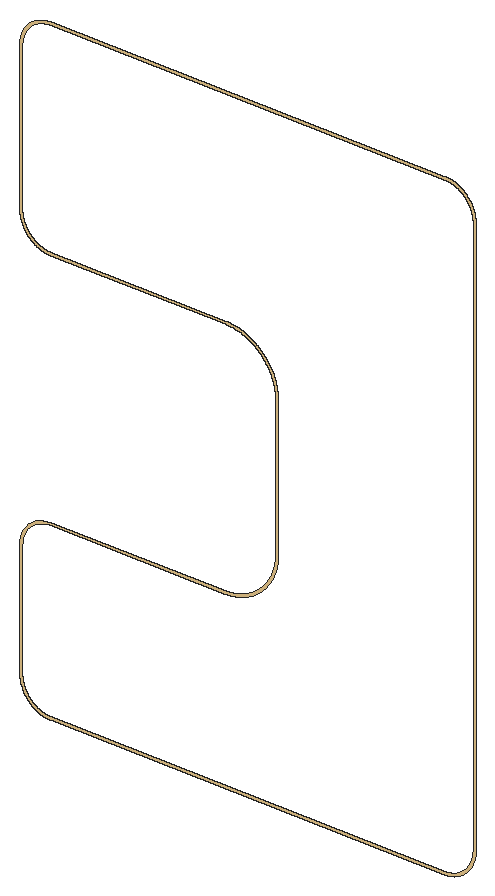
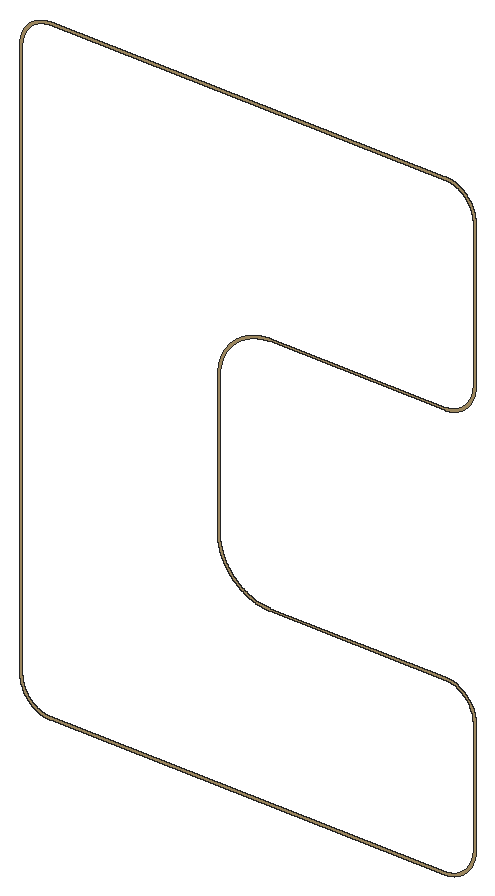
# SketchUp Ruby script. Lengths in inches.
U = 1.inch
M = Sketchup.active_model
def pt(a) = Geom::Point3d.new(a.map { |v| v * U })
def face(e, loops, mat)
  f = e.add_face(loops[0].map { |a| pt(a) })
  loops[1..].each { |l| e.add_face(l.map { |a| pt(a) }).erase! }
  f.material = f.back_material = mat if mat
  f
end
# faces: each face lists its corners as indices into pts; further lists are holes
def faces(e, pts, list, mat = nil) = list.each { |f| face(e, (f[0].is_a?(Array) ? f : [f]).map { |l| l.map { |i| pts[i] } }, mat) }
# xy, xz, yz: faces in a plane at the given z, y or x. An outline is a flat list of corners, or four numbers for a rectangle; further outlines are holes
def ring(l) = l.size == 4 ? [[l[0], l[1]], [l[2], l[1]], [l[2], l[3]], [l[0], l[3]]] : l.each_slice(2).to_a
def flat(e, list, mat, &to3) = list.each { |f| face(e, (f[0].is_a?(Array) ? f : [f]).map { |l| ring(l).map { |u, v| to3.(u, v) } }, mat) }
def xy(e, z, list, mat = nil) = flat(e, list, mat) { |x, y| [x, y, z] }
def xz(e, y, list, mat = nil) = flat(e, list, mat) { |x, z| [x, y, z] }
def yz(e, x, list, mat = nil) = flat(e, list, mat) { |y, z| [x, y, z] }
def lines(e, pts, list) = list.each { |a, b| e.add_line(pt(pts[a]), pt(pts[b])) }
# prism: a flat outline (further loops are holes) pulled along v
def prism(e, loops, v, mat = nil)
  f = face(e, loops, mat); d = Geom::Vector3d.new(v.map { |x| x * U })
  f.pushpull(f.normal.samedirection?(d) ? d.length : -d.length)
end
def box(e, o, s, mat = nil) = prism(e, [[o, [o[0] + s[0], o[1], o[2]], [o[0] + s[0], o[1] + s[1], o[2]], [o[0], o[1] + s[1], o[2]]]], [0, 0, s[2]], mat)
def at(x, y, z, deg = 0) = Geom::Transformation.translation(pt([x, y, z])) * Geom::Transformation.rotation(ORIGIN, Z_AXIS, deg.degrees)
def axes(o, x, y, z) = Geom::Transformation.new([*x, 0, *y, 0, *z, 0, *pt(o).to_a, 1])
def part(name) = M.definitions.add(name)
# library, detail: a bought-in or finely detailed component or shape, given as its bounding box
def library(name, o, s) = part(name).tap { |d| box(d.entities, o, s) }
def detail(e, o, s) = box(e.add_group.entities, o, s)
def put(e, d, t, mat = nil) = e.add_instance(d, t).tap { |i| i.material = mat if mat }
def group(e, t, mat = nil) = e.add_group.tap { |g| g.transformation = t; g.material = mat if mat }.entities
root = M.entities
M.materials.add("Outer Light").color = [251, 217, 152]
xz(root,95.37,[[[278.68,171.29,537.32,171.29,537.48,171.3,537.64,171.3,537.8,171.31,537.97,171.31,538.125,171.32,538.29,171.33,538.45,171.34,538.61,171.36,538.93,171.38,539.25,171.42,539.41,171.43,539.73,171.47,539.89,171.5,540.21,171.54,540.37,171.57,540.52,171.6,540.68,171.625,540.84,171.66,541,171.6875,541.16,171.72,541.31,171.75,541.47,171.79,541.63,171.82,541.79,171.86,541.94,171.9,542.1,171.9375,542.25,171.98,542.41,172.02,542.56,172.0625,542.72,172.11,542.875,172.15,543.03,172.2,543.33,172.3,543.49,172.35,543.94,172.5,544.1,172.56,544.25,172.62,544.4,172.67,544.85,172.85,544.99,172.91,545.14,172.98,545.29,173.04,545.4375,173.11,545.58,173.18,545.73,173.24,545.875,173.3125,546.02,173.38,546.16,173.45,546.31,173.53,546.59,173.67,546.73,173.75,547.02,173.91,547.44,174.15,547.57,174.23,547.71,174.3125,547.85,174.4,547.98,174.48,548.12,174.57,548.25,174.66,548.39,174.75,548.52,174.84,548.66,174.93,548.92,175.11,549.05,175.21,549.18,175.3,549.31,175.4,549.4375,175.5,549.56,175.59,549.82,175.79,549.94,175.89,550.07,176,550.19,176.1,550.3125,176.2,550.4375,176.31,550.56,176.41,550.92,176.74,551.03,176.85,551.27,177.07,551.61,177.41,551.72,177.53,551.83,177.64,551.94,177.76,552.05,177.875,552.16,178,552.27,178.11,552.38,178.24,552.48,178.36,552.59,178.48,552.69,178.6,552.8,178.72,552.9,178.85,553,178.97,553.3,179.36,553.39,179.48,553.49,179.61,553.58,179.74,553.68,179.875,553.77,180,553.86,180.14,553.96,180.27,554.05,180.4,554.13,180.54,554.22,180.67,554.31,180.81,554.39,180.94,554.48,181.08,554.5625,181.22,554.65,181.36,554.89,181.78,554.96,181.92,555.12,182.2,555.19,182.34,555.27,182.49,555.41,182.77,555.48,182.92,555.55,183.0625,555.62,183.21,555.68,183.36,555.75,183.5,555.8125,183.65,555.88,183.8,556.18,184.55,556.23,184.7,556.29,184.85,556.39,185.15,556.45,185.3,556.5,185.46,556.55,185.61,556.59,185.76,556.64,185.92,556.6875,186.07,556.73,186.23,556.77,186.38,556.82,186.54,556.86,186.69,556.9,186.85,556.93,187.01,556.97,187.16,557.01,187.32,557.04,187.48,557.07,187.63,557.11,187.79,557.17,188.11,557.19,188.27,557.25,188.59,557.27,188.74,557.3,188.9,557.32,189.0625,557.34,189.22,557.36,189.38,557.39,189.7,557.41,189.86,557.42,190.02,557.4375,190.18,557.45,190.34,557.46,190.5,557.47,190.67,557.48,190.83,557.48,190.99,557.49,191.15,557.49,191.31,557.5,191.47,557.5,561.11,557.49,561.28,557.49,561.4375,557.48,561.6,557.48,561.76,557.45,562.24,557.4375,562.4,557.42,562.5625,557.41,562.72,557.39,562.88,557.36,563.2,557.3,563.68,557.27,563.84,557.25,564,557.19,564.32,557.17,564.48,557.14,564.63,557.11,564.79,557.07,564.95,557.04,565.11,557.01,565.26,556.93,565.58,556.9,565.73,556.82,566.05,556.77,566.2,556.73,566.36,556.6875,566.51,556.64,566.67,556.59,566.82,556.55,566.97,556.45,567.28,556.39,567.43,556.34,567.58,556.29,567.74,556.23,567.89,556.18,568.04,556.12,568.1875,556.06,568.34,555.88,568.79,555.8125,568.93,555.75,569.08,555.68,569.23,555.62,569.375,555.55,569.52,555.48,569.67,555.41,569.8125,555.34,569.96,555.27,570.1,555.19,570.24,555.12,570.38,555.04,570.53,554.96,570.67,554.89,570.81,554.65,571.23,554.5625,571.37,554.48,571.5,554.39,571.64,554.31,571.78,554.22,571.91,554.13,572.05,554.05,572.18,553.96,572.31,553.86,572.45,553.68,572.71,553.58,572.84,553.49,572.97,553.39,573.1,553.3,573.23,553.2,573.36,553.1,573.48,553,573.61,552.9,573.73,552.8,573.86,552.69,573.98,552.59,574.11,552.48,574.23,552.38,574.35,551.94,574.83,551.83,574.94,551.72,575.06,551.61,575.17,551.5,575.29,551.38,575.4,551.27,575.51,551.03,575.74,550.92,575.85,550.8,575.95,550.68,576.0625,550.56,576.17,550.4375,576.28,550.3125,576.38,550.19,576.48,550.07,576.59,549.94,576.69,549.82,576.79,549.56,576.99,549.4375,577.09,549.31,577.1875,549.18,577.28,548.92,577.47,548.79,577.5625,548.66,577.66,548.52,577.75,548.39,577.84,548.25,577.93,548.12,578.01,547.98,578.1,547.85,578.1875,547.71,578.27,547.57,578.35,547.44,578.4375,547.3,578.52,547.02,578.68,546.875,578.76,546.73,578.83,546.59,578.91,546.45,578.98,546.31,579.06,546.16,579.13,546.02,579.2,545.73,579.34,545.58,579.41,545.4375,579.48,545.29,579.54,545.14,579.61,544.99,579.67,544.85,579.73,544.25,579.97,544.1,580.02,543.94,580.08,543.79,580.13,543.64,580.1875,543.49,580.24,543.33,580.29,543.03,580.39,542.875,580.43,542.72,580.48,542.56,580.52,542.41,580.57,542.25,580.61,542.1,580.65,541.94,580.6875,541.79,580.73,541.63,580.76,541.47,580.8,541.31,580.83,541.16,580.87,540.52,580.99,540.37,581.01,540.21,581.04,540.05,581.0625,539.89,581.09,539.09,581.19,538.93,581.2,538.77,581.22,538.29,581.25,538.125,581.26,537.97,581.27,537.8,581.28,537.64,581.28,537.48,581.29,278.52,581.29,278.36,581.28,278.2,581.28,278.03,581.27,277.875,581.26,277.71,581.25,277.23,581.22,277.07,581.2,276.91,581.19,276.11,581.09,275.95,581.0625,275.79,581.04,275.63,581.01,275.48,580.99,274.84,580.87,274.69,580.83,274.53,580.8,274.37,580.76,274.21,580.73,274.06,580.6875,273.9,580.65,273.75,580.61,273.59,580.57,273.44,580.52,273.28,580.48,273.125,580.43,272.97,580.39,272.67,580.29,272.51,580.24,272.36,580.1875,272.21,580.13,272.06,580.08,271.9,580.02,271.75,579.97,271.15,579.73,271.01,579.67,270.86,579.61,270.71,579.54,270.5625,579.48,270.42,579.41,270.27,579.34,269.98,579.2,269.84,579.13,269.69,579.06,269.55,578.98,269.41,578.91,269.27,578.83,269.125,578.76,268.98,578.68,268.7,578.52,268.56,578.4375,268.43,578.35,268.29,578.27,268.15,578.1875,268.02,578.1,267.88,578.01,267.75,577.93,267.61,577.84,267.48,577.75,267.34,577.66,267.21,577.5625,267.08,577.47,266.82,577.28,266.69,577.1875,266.5625,577.09,266.44,576.99,266.18,576.79,266.06,576.69,265.93,576.59,265.81,576.48,265.6875,576.38,265.5625,576.28,265.44,576.17,265.32,576.0625,265.2,575.95,265.08,575.85,264.97,575.74,264.73,575.51,264.62,575.4,264.5,575.29,264.39,575.17,264.28,575.06,264.17,574.94,264.06,574.83,263.62,574.35,263.52,574.23,263.41,574.11,263.31,573.98,263.2,573.86,263.1,573.73,263,573.61,262.9,573.48,262.8,573.36,262.7,573.23,262.61,573.1,262.51,572.97,262.42,572.84,262.32,572.71,262.14,572.45,262.04,572.31,261.95,572.18,261.87,572.05,261.78,571.91,261.69,571.78,261.61,571.64,261.52,571.5,261.4375,571.37,261.35,571.23,261.11,570.81,261.04,570.67,260.96,570.53,260.88,570.38,260.81,570.24,260.73,570.1,260.66,569.96,260.59,569.8125,260.52,569.67,260.45,569.52,260.38,569.375,260.32,569.23,260.25,569.08,260.1875,568.93,260.12,568.79,259.94,568.34,259.88,568.1875,259.82,568.04,259.77,567.89,259.71,567.74,259.66,567.58,259.61,567.43,259.55,567.28,259.45,566.97,259.41,566.82,259.36,566.67,259.3125,566.51,259.27,566.36,259.23,566.2,259.18,566.05,259.1,565.73,259.07,565.58,258.99,565.26,258.96,565.11,258.93,564.95,258.89,564.79,258.86,564.63,258.83,564.48,258.81,564.32,258.75,564,258.73,563.84,258.7,563.68,258.64,563.2,258.61,562.88,258.59,562.72,258.58,562.5625,258.5625,562.4,258.55,562.24,258.52,561.76,258.52,561.6,258.51,561.4375,258.51,561.28,258.5,561.11,258.5,464.47,258.51,464.31,258.51,464.15,258.52,463.99,258.52,463.83,258.53,463.67,258.54,463.5,258.55,463.34,258.5625,463.18,258.58,463.02,258.59,462.86,258.61,462.7,258.64,462.38,258.66,462.22,258.68,462.0625,258.7,461.9,258.73,461.74,258.75,461.59,258.81,461.27,258.83,461.11,258.89,460.79,258.93,460.63,258.96,460.48,258.99,460.32,259.03,460.16,259.07,460.01,259.1,459.85,259.14,459.69,259.18,459.54,259.23,459.38,259.27,459.23,259.3125,459.07,259.36,458.92,259.41,458.76,259.45,458.61,259.5,458.46,259.55,458.3,259.61,458.15,259.71,457.85,259.77,457.7,259.82,457.55,260.12,456.8,260.1875,456.65,260.25,456.5,260.32,456.36,260.38,456.21,260.45,456.0625,260.52,455.92,260.59,455.77,260.73,455.49,260.81,455.34,260.88,455.2,261.04,454.92,261.11,454.78,261.35,454.36,261.4375,454.22,261.52,454.08,261.61,453.94,261.69,453.81,261.78,453.67,261.87,453.54,261.95,453.4,262.04,453.27,262.14,453.14,262.23,453,262.32,452.875,262.42,452.74,262.51,452.61,262.61,452.48,262.7,452.36,263,451.97,263.1,451.85,263.2,451.72,263.31,451.6,263.41,451.48,263.52,451.36,263.62,451.24,263.73,451.11,263.84,451,263.95,450.875,264.06,450.76,264.17,450.64,264.28,450.53,264.39,450.41,264.73,450.07,264.97,449.85,265.08,449.74,265.44,449.41,265.5625,449.31,265.6875,449.2,265.81,449.1,265.93,449,266.06,448.89,266.18,448.79,266.44,448.59,266.5625,448.5,266.69,448.4,266.82,448.3,266.95,448.21,267.08,448.11,267.34,447.93,267.48,447.84,267.61,447.75,267.75,447.66,267.88,447.57,268.02,447.48,268.15,447.4,268.29,447.3125,268.43,447.23,268.56,447.15,268.98,446.91,269.27,446.75,269.41,446.67,269.69,446.53,269.84,446.45,269.98,446.38,270.125,446.3125,270.27,446.24,270.42,446.18,270.5625,446.11,270.71,446.04,270.86,445.98,271.01,445.91,271.15,445.85,271.6,445.67,271.75,445.62,271.9,445.56,272.06,445.5,272.51,445.35,272.67,445.3,272.97,445.2,273.125,445.15,273.28,445.11,273.44,445.0625,273.59,445.02,273.75,444.98,273.9,444.9375,274.06,444.9,274.21,444.86,274.37,444.82,274.53,444.79,274.69,444.75,274.84,444.72,275,444.6875,275.16,444.66,275.32,444.625,275.48,444.6,275.63,444.57,275.79,444.54,276.11,444.5,276.27,444.47,276.59,444.43,276.75,444.42,277.07,444.38,277.39,444.36,277.55,444.34,277.71,444.33,277.875,444.32,278.03,444.31,278.2,444.31,278.36,444.3,278.52,444.3,278.68,444.29,393.4375,444.29,393.875,444.28,394.32,444.27,394.75,444.25,395.19,444.22,395.63,444.1875,396.07,444.15,396.5,444.11,396.9375,444.06,397.37,444.01,397.81,443.95,398.67,443.81,399.1,443.73,399.54,443.65,399.97,443.56,400.39,443.47,400.82,443.37,401.25,443.26,401.67,443.15,402.93,442.79,403.77,442.51,404.18,442.37,404.59,442.22,405.01,442.07,405.41,441.91,405.82,441.74,406.22,441.57,406.625,441.4,407.03,441.21,407.42,441.03,407.82,440.84,408.21,440.64,408.6,440.4375,408.98,440.23,409.37,440.02,410.13,439.58,410.5,439.36,411.25,438.89,411.61,438.65,412.33,438.15,412.69,437.89,413.39,437.37,413.74,437.1,414.08,436.83,414.76,436.27,415.09,435.98,415.42,435.6875,415.74,435.39,416.06,435.09,416.375,434.79,417,434.17,417.9,433.21,418.1875,432.88,418.47,432.55,418.76,432.21,419.03,431.875,419.31,431.53,419.58,431.1875,419.84,430.84,420.1,430.48,420.36,430.125,420.61,429.77,420.85,429.4,421.1,429.04,421.33,428.67,421.5625,428.3,421.79,427.92,422.23,427.16,422.44,426.78,422.65,426.39,423.05,425.61,423.24,425.21,423.42,424.82,423.78,424.02,423.95,423.61,424.12,423.21,424.27,422.8,424.43,422.39,424.58,421.97,424.72,421.56,424.86,421.14,424.99,420.73,425.12,420.31,425.24,419.89,425.36,419.46,425.47,419.04,425.57,418.61,425.67,418.19,425.77,417.76,425.86,417.33,425.9375,416.9,426.02,416.47,426.09,416.03,426.15,415.6,426.21,415.16,426.27,414.73,426.32,414.29,426.36,413.86,426.4,413.42,426.43,412.98,426.45,412.55,426.49,411.67,426.5,411.23,426.5,320.35,426.49,319.92,426.43,318.6,426.4,318.16,426.36,317.73,426.32,317.29,426.27,316.85,426.15,315.99,426.09,315.55,426.02,315.12,425.9375,314.6875,425.86,314.26,425.77,313.83,425.57,312.97,425.47,312.55,425.36,312.12,425.12,311.28,424.86,310.44,424.72,310.02,424.58,309.61,424.43,309.2,424.27,308.79,424.12,308.38,423.95,307.97,423.78,307.57,423.24,306.37,423.05,305.98,422.85,305.58,422.65,305.19,422.44,304.81,422.23,304.42,421.79,303.66,421.5625,303.29,421.33,302.92,421.1,302.55,420.85,302.18,420.61,301.82,420.36,301.46,420.1,301.1,419.58,300.4,419.31,300.05,419.03,299.71,418.76,299.37,418.47,299.04,418.1875,298.7,417.9,298.375,417.6,298.05,417.3,297.73,417,297.42,416.6875,297.1,416.375,296.8,416.06,296.49,415.74,296.19,415.42,295.9,414.76,295.32,413.74,294.48,413.39,294.21,412.69,293.69,412.33,293.43,411.97,293.18,411.61,292.9375,411.25,292.7,410.875,292.46,410.5,292.23,410.13,292,409.75,291.78,409.37,291.5625,408.98,291.35,408.6,291.14,408.21,290.94,407.82,290.75,407.42,290.56,407.03,290.37,406.625,290.1875,406.22,290.01,405.82,289.84,405.41,289.68,405.01,289.52,404.59,289.36,404.18,289.21,403.77,289.07,403.35,288.93,402.51,288.67,401.67,288.43,401.25,288.32,400.39,288.12,399.97,288.02,399.54,287.9375,399.1,287.85,398.67,287.78,398.24,287.7,397.81,287.64,397.37,287.58,396.9375,287.52,396.5,287.48,396.07,287.43,395.63,287.4,395.19,287.36,394.75,287.34,394.32,287.32,393.875,287.3,393.4375,287.29,279,287.29,276.32,287.12,273.69,286.59,271.15,285.73,268.75,284.55,266.52,283.06,264.5,281.29,262.74,279.27,261.25,277.04,260.06,274.64,259.2,272.1,258.68,269.47,258.5,266.79,258.5,191.47,258.51,191.31,258.51,191.15,258.52,190.99,258.52,190.83,258.53,190.67,258.54,190.5,258.55,190.34,258.5625,190.18,258.58,190.02,258.59,189.86,258.61,189.7,258.64,189.38,258.66,189.22,258.68,189.0625,258.7,188.9,258.73,188.74,258.75,188.59,258.81,188.27,258.83,188.11,258.89,187.79,258.93,187.63,258.96,187.48,258.99,187.32,259.03,187.16,259.07,187.01,259.1,186.85,259.14,186.69,259.18,186.54,259.23,186.38,259.27,186.23,259.3125,186.07,259.36,185.92,259.41,185.76,259.45,185.61,259.5,185.46,259.55,185.3,259.61,185.15,259.71,184.85,259.77,184.7,259.82,184.55,260.12,183.8,260.1875,183.65,260.25,183.5,260.32,183.36,260.38,183.21,260.45,183.0625,260.52,182.92,260.59,182.77,260.73,182.49,260.81,182.34,260.88,182.2,261.04,181.92,261.11,181.78,261.35,181.36,261.4375,181.22,261.52,181.08,261.61,180.94,261.69,180.81,261.78,180.67,261.87,180.54,261.95,180.4,262.04,180.27,262.14,180.14,262.23,180,262.32,179.875,262.42,179.74,262.51,179.61,262.61,179.48,262.7,179.36,263,178.97,263.1,178.85,263.2,178.72,263.31,178.6,263.41,178.48,263.52,178.36,263.62,178.24,263.73,178.11,263.84,178,263.95,177.875,264.06,177.76,264.17,177.64,264.28,177.53,264.39,177.41,264.73,177.07,264.97,176.85,265.08,176.74,265.44,176.41,265.5625,176.31,265.6875,176.2,265.81,176.1,265.93,176,266.06,175.89,266.18,175.79,266.44,175.59,266.5625,175.5,266.69,175.4,266.82,175.3,266.95,175.21,267.08,175.11,267.34,174.93,267.48,174.84,267.61,174.75,267.75,174.66,267.88,174.57,268.02,174.48,268.15,174.4,268.29,174.3125,268.43,174.23,268.56,174.15,268.98,173.91,269.27,173.75,269.41,173.67,269.69,173.53,269.84,173.45,269.98,173.38,270.125,173.3125,270.27,173.24,270.42,173.18,270.5625,173.11,270.71,173.04,270.86,172.98,271.01,172.91,271.15,172.85,271.6,172.67,271.75,172.62,271.9,172.56,272.06,172.5,272.51,172.35,272.67,172.3,272.97,172.2,273.125,172.15,273.28,172.11,273.44,172.0625,273.59,172.02,273.75,171.98,273.9,171.9375,274.06,171.9,274.21,171.86,274.37,171.82,274.53,171.79,274.69,171.75,274.84,171.72,275,171.6875,275.16,171.66,275.32,171.625,275.48,171.6,275.63,171.57,275.79,171.54,276.11,171.5,276.27,171.47,276.59,171.43,276.75,171.42,277.07,171.38,277.39,171.36,277.55,171.34,277.71,171.33,277.875,171.32,278.03,171.31,278.2,171.31,278.36,171.3,278.52,171.3],[278.7,172.79,278.55,172.8,278.4,172.8,278.25,172.81,278.1,172.8125,277.96,172.82,277.36,172.86,277.21,172.875,277.0625,172.89,276.92,172.91,276.77,172.92,276.32,172.98,276.18,173,276.03,173.03,275.73,173.07,275.59,173.1,275.29,173.16,275.15,173.1875,275,173.22,274.86,173.25,274.71,173.28,274.56,173.32,274.42,173.35,274.27,173.39,273.99,173.47,273.84,173.51,273.56,173.59,273.41,173.63,273.27,173.68,273.13,173.72,272.85,173.82,272.7,173.87,272.5625,173.92,272.42,173.97,272.14,174.07,272.01,174.125,271.87,174.18,271.59,174.3,271.45,174.35,271.32,174.41,271.18,174.48,271.05,174.54,270.91,174.6,270.78,174.66,270.64,174.73,270.51,174.8,270.375,174.86,270.24,174.93,269.72,175.21,269.59,175.29,269.46,175.36,269.33,175.4375,269.2,175.51,269.07,175.59,268.95,175.67,268.69,175.83,268.57,175.91,268.44,175.99,268.32,176.08,268.2,176.16,268.07,176.25,267.95,176.33,267.59,176.6,267.47,176.6875,267.35,176.78,267.24,176.87,267.12,176.96,267,177.06,266.89,177.15,266.77,177.25,266.66,177.34,266.44,177.54,266.32,177.64,265.99,177.94,265.78,178.15,265.67,178.25,265.46,178.46,265.36,178.57,265.25,178.68,265.15,178.79,265.05,178.89,264.95,179,264.85,179.12,264.55,179.45,264.46,179.57,264.36,179.68,264.27,179.8,264.17,179.91,263.9,180.27,263.81,180.38,263.72,180.5,263.54,180.75,263.46,180.87,263.37,180.99,263.29,181.11,263.2,181.24,263.12,181.36,263.04,181.49,262.96,181.61,262.88,181.74,262.8,181.86,262.72,181.99,262.65,182.12,262.57,182.25,262.5,182.38,262.42,182.51,262.14,183.03,262.07,183.17,262,183.3,261.9375,183.43,261.87,183.57,261.81,183.7,261.75,183.84,261.68,183.97,261.62,184.11,261.5625,184.25,261.5,184.38,261.45,184.52,261.33,184.8,261.28,184.9375,261.23,185.08,261.17,185.22,261.125,185.36,261.07,185.5,261.02,185.64,260.98,185.78,260.93,185.92,260.88,186.0625,260.84,186.21,260.8,186.35,260.75,186.49,260.71,186.63,260.67,186.78,260.63,186.92,260.6,187.07,260.56,187.21,260.52,187.36,260.49,187.5,260.46,187.65,260.43,187.79,260.39,187.9375,260.37,188.09,260.34,188.23,260.28,188.53,260.26,188.67,260.23,188.82,260.21,188.97,260.19,189.11,260.11,189.71,260.1,189.86,260.08,190,260.01,191.05,260.01,191.34,260,191.49,260,266.79,260.16,269.27,260.65,271.71,261.45,274.0625,262.55,276.29,263.93,278.36,265.56,280.23,267.43,281.87,269.5,283.25,271.73,284.35,274.08,285.14,276.52,285.63,279,285.79,393,285.79,393.46,285.8,393.92,285.8,394.83,285.84,395.75,285.9,396.2,285.9375,396.66,285.98,397.11,286.03,397.57,286.09,398.02,286.15,398.48,286.22,399.83,286.46,400.28,286.56,400.72,286.66,401.17,286.76,401.62,286.87,402.06,286.98,402.5,287.11,402.94,287.23,403.82,287.51,404.25,287.65,404.68,287.8,405.97,288.28,406.39,288.46,406.82,288.63,407.24,288.82,407.65,289.01,408.07,289.2,408.48,289.4,409.3,289.82,409.7,290.03,410.1,290.25,410.9,290.71,411.68,291.19,412.0625,291.4375,412.44,291.69,413.2,292.21,414.31,293.02,414.67,293.31,415.03,293.59,415.38,293.88,416.08,294.48,416.42,294.78,416.76,295.09,417.09,295.4,417.75,296.04,418.39,296.7,418.7,297.03,419.01,297.37,419.3125,297.71,419.61,298.0625,419.91,298.41,420.2,298.77,420.49,299.125,420.77,299.49,421.04,299.85,421.32,300.22,421.58,300.59,422.1,301.35,422.35,301.73,422.6,302.12,422.84,302.5,423.08,302.9,423.3125,303.29,423.54,303.69,423.76,304.09,423.97,304.5,424.19,304.9,424.39,305.3125,424.59,305.72,424.79,306.14,424.97,306.56,425.16,306.98,425.34,307.4,425.51,307.82,425.68,308.25,425.84,308.68,426.14,309.54,426.29,309.98,426.43,310.41,426.56,310.85,426.6875,311.29,426.81,311.73,426.92,312.18,427.03,312.62,427.14,313.07,427.24,313.52,427.33,313.96,427.49,314.86,427.57,315.32,427.64,315.77,427.7,316.22,427.76,316.68,427.81,317.13,427.89,318.05,427.93,318.5,427.97,319.42,427.99,319.875,428,320.33,428,411.25,427.99,411.71,427.97,412.17,427.93,413.08,427.89,413.54,427.85,413.99,427.81,414.45,427.76,414.91,427.7,415.36,427.64,415.8125,427.57,416.27,427.33,417.62,427.24,418.07,427.14,418.52,427.03,418.96,426.92,419.41,426.81,419.85,426.6875,420.29,426.56,420.73,426.43,421.17,426.29,421.61,426.14,422.04,425.99,422.48,425.84,422.91,425.68,423.33,425.51,423.76,425.34,424.1875,425.16,424.61,424.97,425.03,424.79,425.45,424.19,426.68,423.97,427.09,423.76,427.49,423.54,427.89,423.3125,428.29,423.08,428.6875,422.84,429.08,422.6,429.47,422.35,429.85,422.1,430.24,421.84,430.62,421.32,431.36,421.04,431.73,420.77,432.1,420.49,432.46,420.2,432.82,419.91,433.17,419.61,433.52,419.3125,433.87,419.01,434.21,418.7,434.55,418.39,434.88,417.75,435.54,417.09,436.18,416.76,436.49,416.08,437.11,415.73,437.41,415.03,437.99,414.67,438.28,414.31,438.56,413.94,438.84,413.57,439.11,413.2,439.375,412.82,439.64,412.44,439.89,412.0625,440.15,411.68,440.39,410.9,440.87,410.1,441.33,409.3,441.77,408.89,441.98,408.07,442.38,407.65,442.58,407.24,442.77,406.82,442.95,406.39,443.13,405.97,443.3,405.54,443.47,405.11,443.63,403.82,444.08,403.38,444.22,402.5,444.48,401.62,444.72,401.17,444.82,400.72,444.93,400.28,445.03,399.38,445.21,398.93,445.29,398.48,445.36,398.02,445.43,397.57,445.49,397.11,445.55,396.66,445.6,396.2,445.65,395.75,445.68,395.29,445.72,394.83,445.74,394.375,445.77,393.92,445.78,393.46,445.79,278.7,445.79,278.55,445.8,278.4,445.8,278.25,445.81,278.1,445.8125,277.96,445.82,277.36,445.86,277.21,445.875,277.0625,445.89,276.92,445.91,276.77,445.92,276.32,445.98,276.18,446,276.03,446.03,275.73,446.07,275.59,446.1,275.29,446.16,275.15,446.1875,275,446.22,274.86,446.25,274.71,446.28,274.56,446.32,274.42,446.35,274.27,446.39,273.99,446.47,273.84,446.51,273.56,446.59,273.41,446.63,273.27,446.68,273.13,446.72,272.85,446.82,272.7,446.87,272.5625,446.92,272.42,446.97,272.14,447.07,272.01,447.125,271.87,447.18,271.59,447.3,271.45,447.35,271.32,447.41,271.18,447.48,271.05,447.54,270.91,447.6,270.78,447.66,270.64,447.73,270.51,447.8,270.375,447.86,270.24,447.93,269.72,448.21,269.59,448.29,269.46,448.36,269.33,448.4375,269.2,448.51,269.07,448.59,268.95,448.67,268.69,448.83,268.57,448.91,268.44,448.99,268.32,449.08,268.2,449.16,268.07,449.25,267.95,449.33,267.59,449.6,267.47,449.6875,267.35,449.78,267.24,449.87,267.12,449.96,267,450.06,266.89,450.15,266.77,450.25,266.66,450.34,266.44,450.54,266.32,450.64,265.99,450.94,265.78,451.15,265.67,451.25,265.46,451.46,265.36,451.57,265.25,451.68,265.15,451.79,265.05,451.89,264.95,452,264.85,452.12,264.55,452.45,264.46,452.57,264.36,452.68,264.27,452.8,264.17,452.91,263.9,453.27,263.81,453.38,263.72,453.5,263.54,453.75,263.46,453.87,263.37,453.99,263.29,454.11,263.2,454.24,263.12,454.36,263.04,454.49,262.96,454.61,262.88,454.74,262.8,454.86,262.72,454.99,262.65,455.12,262.57,455.25,262.5,455.38,262.42,455.51,262.14,456.03,262.07,456.17,262,456.3,261.9375,456.43,261.87,456.57,261.81,456.7,261.75,456.84,261.68,456.97,261.62,457.11,261.5625,457.25,261.5,457.38,261.45,457.52,261.33,457.8,261.28,457.9375,261.23,458.08,261.17,458.22,261.125,458.36,261.07,458.5,261.02,458.64,260.98,458.78,260.93,458.92,260.88,459.0625,260.84,459.21,260.8,459.35,260.75,459.49,260.71,459.63,260.67,459.78,260.63,459.92,260.6,460.07,260.56,460.21,260.52,460.36,260.49,460.5,260.46,460.65,260.43,460.79,260.39,460.9375,260.37,461.09,260.34,461.23,260.28,461.53,260.26,461.67,260.23,461.82,260.21,461.97,260.19,462.11,260.11,462.71,260.1,462.86,260.08,463,260.01,464.05,260.01,464.34,260,464.49,260,561.09,260.01,561.24,260.01,561.54,260.02,561.6875,260.03,561.84,260.04,561.99,260.05,562.13,260.08,562.58,260.1,562.73,260.11,562.88,260.13,563.03,260.15,563.17,260.21,563.62,260.23,563.76,260.26,563.91,260.28,564.06,260.31,564.21,260.34,564.35,260.37,564.5,260.39,564.65,260.43,564.79,260.46,564.9375,260.49,565.08,260.52,565.23,260.56,565.37,260.6,565.52,260.63,565.66,260.67,565.81,260.75,566.09,260.8,566.24,260.88,566.52,260.93,566.66,260.98,566.81,261.02,566.95,261.07,567.09,261.125,567.23,261.17,567.37,261.23,567.51,261.33,567.79,261.39,567.92,261.45,568.0625,261.5,568.2,261.5625,568.34,261.62,568.47,261.68,568.61,261.75,568.75,261.81,568.88,261.87,569.02,261.9375,569.15,262,569.28,262.07,569.42,262.21,569.68,262.28,569.8125,262.35,569.95,262.42,570.08,262.5,570.21,262.57,570.34,262.65,570.46,262.72,570.59,262.88,570.85,262.96,570.97,263.04,571.1,263.12,571.22,263.2,571.35,263.29,571.47,263.37,571.59,263.46,571.72,263.54,571.84,263.9,572.32,263.99,572.4375,264.08,572.55,264.17,572.67,264.27,572.79,264.36,572.9,264.46,573.02,264.55,573.13,264.65,573.24,264.75,573.36,264.95,573.58,265.05,573.6875,265.15,573.8,265.25,573.91,265.36,574.01,265.56,574.23,265.67,574.33,265.78,574.4375,265.89,574.54,265.99,574.64,266.1,574.74,266.21,574.85,266.32,574.95,266.44,575.04,266.77,575.34,266.89,575.43,267,575.53,267.24,575.71,267.35,575.8,267.47,575.9,267.71,576.08,267.83,576.16,268.07,576.34,268.2,576.42,268.32,576.51,268.44,576.59,268.57,576.67,268.69,576.75,268.95,576.91,269.07,576.99,269.33,577.15,269.46,577.22,269.59,577.3,270.24,577.65,270.51,577.79,270.64,577.85,270.78,577.92,270.91,577.98,271.05,578.05,271.18,578.11,271.32,578.17,271.45,578.23,271.73,578.35,271.87,578.4,272.01,578.46,272.14,578.51,272.28,578.57,272.42,578.62,272.5625,578.67,272.7,578.72,272.85,578.77,272.99,578.82,273.13,578.86,273.27,578.91,273.41,578.95,273.56,579,273.84,579.08,273.99,579.12,274.27,579.2,274.42,579.23,274.56,579.27,274.86,579.33,275,579.37,275.15,579.4,275.29,579.43,275.44,579.46,275.59,579.48,275.73,579.51,275.88,579.53,276.03,579.56,276.18,579.58,276.32,579.6,276.92,579.68,277.0625,579.69,277.21,579.71,277.96,579.76,278.1,579.77,278.25,579.78,278.4,579.78,278.55,579.79,537.45,579.79,537.6,579.78,537.75,579.78,537.9,579.77,538.04,579.76,538.79,579.71,538.9375,579.69,539.08,579.68,539.68,579.6,539.82,579.58,539.97,579.56,540.12,579.53,540.27,579.51,540.41,579.48,540.56,579.46,540.71,579.43,540.85,579.4,541,579.37,541.14,579.33,541.44,579.27,541.58,579.23,541.73,579.2,542.01,579.12,542.16,579.08,542.44,579,542.59,578.95,542.73,578.91,542.87,578.86,543.01,578.82,543.15,578.77,543.3,578.72,543.4375,578.67,543.58,578.62,543.72,578.57,543.86,578.51,543.99,578.46,544.13,578.4,544.27,578.35,544.55,578.23,544.68,578.17,544.82,578.11,544.95,578.05,545.09,577.98,545.22,577.92,545.36,577.85,545.49,577.79,545.76,577.65,546.41,577.3,546.54,577.22,546.67,577.15,546.93,576.99,547.05,576.91,547.31,576.75,547.43,576.67,547.56,576.59,547.68,576.51,547.8,576.42,547.93,576.34,548.17,576.16,548.29,576.08,548.53,575.9,548.65,575.8,548.76,575.71,549,575.53,549.11,575.43,549.23,575.34,549.56,575.04,549.68,574.95,549.79,574.85,549.9,574.74,550.01,574.64,550.11,574.54,550.22,574.4375,550.33,574.33,550.44,574.23,550.64,574.01,550.75,573.91,550.85,573.8,550.95,573.6875,551.05,573.58,551.25,573.36,551.35,573.24,551.45,573.13,551.54,573.02,551.64,572.9,551.73,572.79,551.83,572.67,551.92,572.55,552.01,572.4375,552.1,572.32,552.46,571.84,552.54,571.72,552.63,571.59,552.71,571.47,552.8,571.35,552.88,571.22,552.96,571.1,553.04,570.97,553.12,570.85,553.28,570.59,553.35,570.46,553.43,570.34,553.5,570.21,553.58,570.08,553.65,569.95,553.72,569.8125,553.79,569.68,553.93,569.42,554,569.28,554.0625,569.15,554.13,569.02,554.19,568.88,554.25,568.75,554.32,568.61,554.38,568.47,554.4375,568.34,554.5,568.2,554.55,568.0625,554.61,567.92,554.67,567.79,554.77,567.51,554.83,567.37,554.875,567.23,554.93,567.09,554.98,566.95,555.02,566.81,555.07,566.66,555.12,566.52,555.2,566.24,555.25,566.09,555.33,565.81,555.37,565.66,555.4,565.52,555.44,565.37,555.48,565.23,555.51,565.08,555.54,564.9375,555.57,564.79,555.61,564.65,555.63,564.5,555.66,564.35,555.69,564.21,555.72,564.06,555.74,563.91,555.77,563.76,555.79,563.62,555.85,563.17,555.87,563.03,555.89,562.88,555.9,562.73,555.92,562.58,555.95,562.13,555.96,561.99,555.97,561.84,555.98,561.6875,555.99,561.54,555.99,561.24,556,561.09,556,191.49,555.99,191.34,555.99,191.05,555.92,190,555.9,189.86,555.89,189.71,555.81,189.11,555.79,188.97,555.77,188.82,555.74,188.67,555.72,188.53,555.66,188.23,555.63,188.09,555.61,187.9375,555.57,187.79,555.54,187.65,555.51,187.5,555.48,187.36,555.44,187.21,555.4,187.07,555.37,186.92,555.33,186.78,555.29,186.63,555.25,186.49,555.2,186.35,555.16,186.21,555.12,186.0625,555.07,185.92,555.02,185.78,554.98,185.64,554.93,185.5,554.875,185.36,554.83,185.22,554.77,185.08,554.72,184.9375,554.67,184.8,554.55,184.52,554.5,184.38,554.4375,184.25,554.38,184.11,554.32,183.97,554.25,183.84,554.19,183.7,554.13,183.57,554.0625,183.43,554,183.3,553.93,183.17,553.86,183.03,553.58,182.51,553.5,182.38,553.43,182.25,553.35,182.12,553.28,181.99,553.2,181.86,553.12,181.74,553.04,181.61,552.96,181.49,552.88,181.36,552.8,181.24,552.71,181.11,552.63,180.99,552.54,180.87,552.46,180.75,552.28,180.5,552.19,180.38,552.1,180.27,551.83,179.91,551.73,179.8,551.64,179.68,551.54,179.57,551.45,179.45,551.15,179.12,551.05,179,550.95,178.89,550.85,178.79,550.75,178.68,550.64,178.57,550.54,178.46,550.33,178.25,550.22,178.15,550.01,177.94,549.68,177.64,549.56,177.54,549.34,177.34,549.23,177.25,549.11,177.15,549,177.06,548.88,176.96,548.76,176.87,548.65,176.78,548.53,176.6875,548.41,176.6,548.05,176.33,547.93,176.25,547.8,176.16,547.68,176.08,547.56,175.99,547.43,175.91,547.31,175.83,547.05,175.67,546.93,175.59,546.8,175.51,546.67,175.4375,546.54,175.36,546.41,175.29,546.28,175.21,545.76,174.93,545.625,174.86,545.49,174.8,545.36,174.73,545.22,174.66,545.09,174.6,544.95,174.54,544.82,174.48,544.68,174.41,544.55,174.35,544.41,174.3,544.13,174.18,543.99,174.125,543.86,174.07,543.58,173.97,543.4375,173.92,543.3,173.87,543.15,173.82,542.87,173.72,542.73,173.68,542.59,173.63,542.44,173.59,542.16,173.51,542.01,173.47,541.73,173.39,541.58,173.35,541.44,173.32,541.29,173.28,541.14,173.25,541,173.22,540.85,173.1875,540.71,173.16,540.41,173.1,540.27,173.07,539.97,173.03,539.82,173,539.68,172.98,539.23,172.92,539.08,172.91,538.9375,172.89,538.79,172.875,538.64,172.86,538.04,172.82,537.9,172.8125,537.75,172.81,537.6,172.8,537.45,172.8,537.3,172.79]]],"Outer Light")
